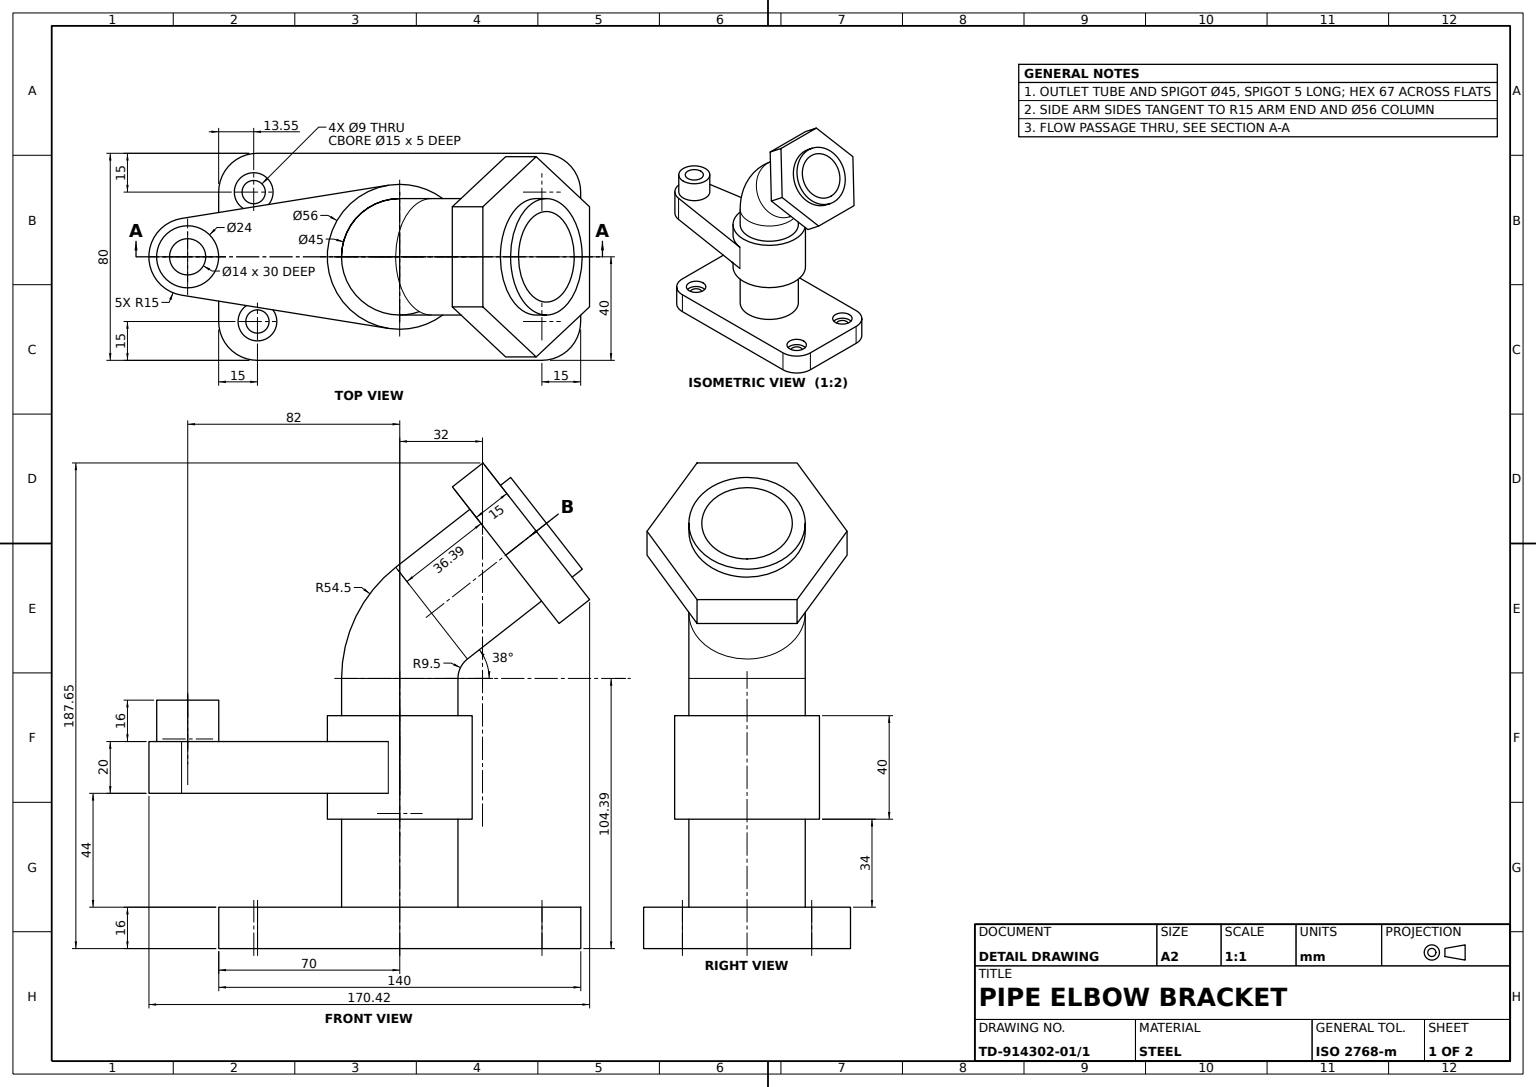
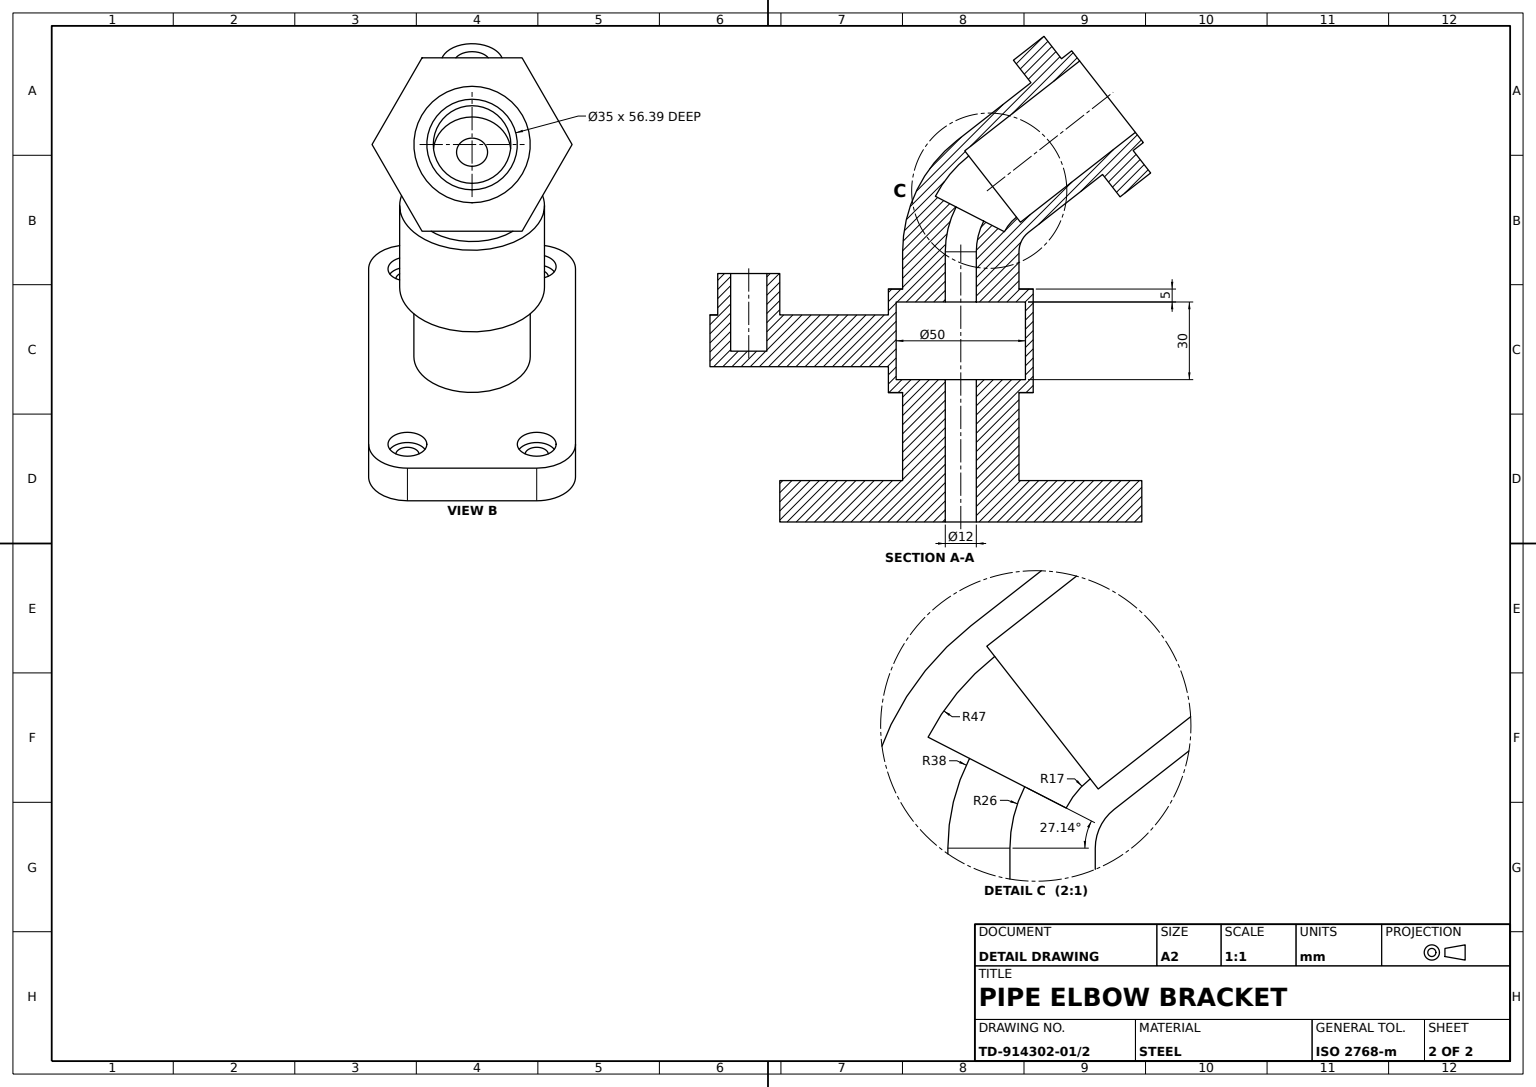
solid
v1 (-55,11,17.5)
v2 (-55,16,17.5)
e1 v1 v2 LINE
v3 (-55,16,32.5)
e2 v2 v3 CIRCLE(AX(P(-55,16,25),D(0,1,0),D(0,0,1)),7.5)
v4 (-55,11,32.5)
e3 v4 v3 LINE
e4 v1 v4 CIRCLE(AX(P(-55,11,25),D(0,1,0),D(0,0,1)),7.5)
face CYL(AX(P(-55,16,25),D(0,1,0),D(0,0,1)),7.5) rev [e1 e2 -e3 -e4]
v5 (61.601219,125.616036,19.341234)
v6 (73.42138,134.850959,19.341234)
e5 v5 v6 LINE
v7 (61.601219,125.616036,-19.341234)
e6 v5 v7 LINE
v8 (73.42138,134.850959,-19.341234)
e7 v7 v8 LINE
e8 v6 v8 LINE
face PLANE(AX(P(61.601219,125.616036,19.341234),D(0.615661475,-0.788010754,0),D(0.788010754,0.615661475,0))) [-e5 e6 e7 -e8]
v9 (-82,80,-12)
v10 (-82,80,12)
e9 v9 v10 CIRCLE(AX(P(-82,80,0),D(0,1,0),D(0,0,1)),12)
v11 (-82,96,12)
e10 v11 v10 LINE
v12 (-82,96,-12)
e11 v12 v11 CIRCLE(AX(P(-82,96,0),D(0,1,0),D(0,0,1)),12)
e12 v12 v9 LINE
face CYL(AX(P(-82,96,0),D(0,-1,0),D(0,0,-1)),12) [e9 -e10 -e11 e12]
v13 (55,11,17.5)
v14 (55,16,17.5)
e13 v13 v14 LINE
v15 (55,11,32.5)
e14 v15 v13 CIRCLE(AX(P(55,11,25),D(0,1,0),D(0,0,1)),7.5)
v16 (55,16,32.5)
e15 v15 v16 LINE
e16 v16 v14 CIRCLE(AX(P(55,16,25),D(0,1,0),D(0,0,1)),7.5)
face CYL(AX(P(55,16,25),D(0,1,0),D(0,0,1)),7.5) rev [-e13 -e14 e15 e16]
v17 (0,90,22.5)
v18 (0,90,-22.5)
e17 v17 v18 CIRCLE(AX(P(0,90,0),D(0,-1,0),D(0,0,1)),22.5)
v19 (0,104.392557,22.5)
e18 v17 v19 LINE
v20 (-22.5,104.392557,0)
e19 v19 v20 CIRCLE(AX(P(0,104.392557,0),D(0,-1,0),D(1,0,0)),22.5)
v21 (0,104.392557,-22.5)
e20 v20 v21 CIRCLE(AX(P(0,104.392557,0),D(0,-1,0),D(1,0,0)),22.5)
e21 v18 v21 LINE
face CYL(AX(P(0,0,0),D(0,1,0),D(0,0,1)),22.5) [-e17 e18 e19 e20 -e21]
v22 (0,0,6)
v23 (0,0,-6)
e22 v22 v23 CIRCLE(AX(P(0,0,0),D(0,-1,0),D(0,0,-1)),6)
v24 (0,55,-6)
e23 v23 v24 LINE
v25 (0,55,6)
e24 v24 v25 CIRCLE(AX(P(0,55,0),D(0,1,0),D(0,0,1)),6)
e25 v22 v25 LINE
face CYL(AX(P(0,-1.043926,0),D(0,1,0),D(0,0,1)),6) rev [e22 e23 e24 -e25]
v26 (27.124176,169.744639,0)
v27 (54.828942,134.284155,0)
e26 v26 v27 CIRCLE(AX(P(40.976559,152.014397,0),D(0.788010754,0.615661475,0),D(-0.615661475,0.788010754,0)),22.5)
e27 v27 v26 CIRCLE(AX(P(40.976559,152.014397,0),D(0.788010754,0.615661475,0),D(-0.615661475,0.788010754,0)),22.5)
v28 (20.3519,178.412757,19.341234)
v29 (40.976559,152.014397,38.682468)
e28 v28 v29 LINE
v30 (20.3519,178.412757,-19.341234)
e29 v30 v28 LINE
v31 (40.976559,152.014397,-38.682468)
e30 v31 v30 LINE
e31 v7 v31 LINE
e32 v29 v5 LINE
face PLANE(AX(P(99.194303,77.499083,0),D(0.788010754,0.615661475,0),D(-0.615661475,0.788010754,0))) rev [e26 e27] [-e28 -e29 -e30 -e31 -e6 -e32]
v32 (70,16,25)
v33 (70,16,-25)
e33 v32 v33 LINE
v34 (70,0,25)
e34 v32 v34 LINE
v35 (70,0,-25)
e35 v34 v35 LINE
e36 v35 v33 LINE
face PLANE(AX(P(70,16,40),D(-1,0,0),D(0,0,1))) rev [-e33 e34 e35 e36]
v36 (-56.445631,0,-29.5)
v37 (-56.445631,11,-29.5)
e37 v36 v37 LINE
v38 (-56.445631,0,-20.5)
e38 v36 v38 CIRCLE(AX(P(-56.445631,0,-25),D(0,-1,0),D(0,0,-1)),4.5)
v39 (-56.445631,11,-20.5)
e39 v38 v39 LINE
e40 v39 v37 CIRCLE(AX(P(-56.445631,11,-25),D(0,1,0),D(0,0,1)),4.5)
face CYL(AX(P(-56.445631,16,-25),D(0,1,0),D(0,0,1)),4.5) rev [-e37 e38 e39 e40]
v40 (52.79672,161.249319,38.682468)
e41 v40 v6 LINE
e42 v29 v40 LINE
face PLANE(AX(P(40.976559,152.014397,38.682468),D(0.307830738,-0.394005377,0.866025404),D(0,-0.91022489,-0.414114296))) [e5 -e41 -e42 e32]
v41 (55,11,29.5)
v42 (55,11,20.5)
e43 v41 v42 CIRCLE(AX(P(55,11,25),D(0,1,0),D(0,0,1)),4.5)
e44 v42 v41 CIRCLE(AX(P(55,11,25),D(0,1,0),D(0,0,1)),4.5)
e45 v13 v15 CIRCLE(AX(P(55,11,25),D(0,1,0),D(0,0,1)),7.5)
face PLANE(AX(P(59.5,11,25),D(0,-1,0),D(0,0,-1))) rev [-e43 -e44] [e45 e14]
v43 (-84.378049,60,14.810297)
v44 (-4.439024,60,27.645887)
e46 v43 v44 LINE
v45 (-84.378049,60,-14.810297)
e47 v45 v43 CIRCLE(AX(P(-82,60,0),D(0,1,0),D(0,0,1)),15)
v46 (-4.439024,60,-27.645887)
e48 v46 v45 LINE
e49 v44 v46 CIRCLE(AX(P(0,60,0),D(0,-1,0),D(0,0,1)),28)
face PLANE(AX(P(-82,60,0),D(0,1,0),D(0,0,1))) rev [-e46 -e47 -e48 -e49]
v47 (55,11,-17.5)
v48 (55,16,-17.5)
e50 v47 v48 LINE
v49 (55,16,-32.5)
e51 v48 v49 CIRCLE(AX(P(55,16,-25),D(0,1,0),D(0,0,1)),7.5)
v50 (55,11,-32.5)
e52 v50 v49 LINE
e53 v47 v50 CIRCLE(AX(P(55,11,-25),D(0,1,0),D(0,0,1)),7.5)
face CYL(AX(P(55,16,-25),D(0,1,0),D(0,0,1)),7.5) rev [e50 e51 -e52 -e53]
v51 (55,16,40)
e54 v51 v32 CIRCLE(AX(P(55,16,25),D(0,1,0),D(0,0,-1)),15)
v52 (55,0,40)
e55 v52 v51 LINE
e56 v34 v52 CIRCLE(AX(P(55,0,25),D(0,-1,0),D(0,0,-1)),15)
face CYL(AX(P(55,16,25),D(0,-1,0),D(0,0,-1)),15) [-e54 -e55 -e56 -e34]
v53 (0,55,-25)
v54 (0,55,25)
e57 v53 v54 CIRCLE(AX(P(0,55,0),D(0,-1,0),D(0,0,-1)),25)
e58 v54 v53 CIRCLE(AX(P(0,55,0),D(0,-1,0),D(0,0,-1)),25)
e59 v25 v24 CIRCLE(AX(P(0,55,0),D(0,1,0),D(0,0,1)),6)
face PLANE(AX(P(-25,55,0),D(0,1,0),D(0,0,1))) [-e57 -e58] [-e24 -e59]
e60 v10 v9 CIRCLE(AX(P(-82,80,0),D(0,1,0),D(0,0,1)),12)
e61 v11 v12 CIRCLE(AX(P(-82,96,0),D(0,1,0),D(0,0,1)),12)
face CYL(AX(P(-82,96,0),D(0,-1,0),D(0,0,-1)),12) [e10 e60 -e12 -e61]
v55 (-4.439024,80,27.645887)
v56 (-4.439024,80,-27.645887)
e62 v55 v56 CIRCLE(AX(P(0,80,0),D(0,-1,0),D(0,0,1)),28)
e63 v55 v44 LINE
e64 v56 v46 LINE
v57 (0,90,28)
v58 (0,50,28)
e65 v57 v58 LINE
v59 (0,90,-28)
e66 v59 v57 CIRCLE(AX(P(0,90,0),D(0,1,0),D(0,0,1)),28)
v60 (0,50,-28)
e67 v59 v60 LINE
e68 v60 v58 CIRCLE(AX(P(0,50,0),D(0,1,0),D(0,0,1)),28)
face CYL(AX(P(0,90,0),D(0,-1,0),D(0,0,-1)),28) [-e62 e63 e49 -e64] [-e65 -e66 e67 e68]
v61 (-84.378049,80,-14.810297)
e69 v56 v61 LINE
e70 v61 v45 LINE
face PLANE(AX(P(-84.378049,80,-14.810297),D(0.158536585,0,0.987353104),D(0.987353104,0,-0.158536585))) rev [-e69 e64 e48 -e70]
v62 (0,85,25)
v63 (0,85,-25)
e71 v62 v63 CIRCLE(AX(P(0,85,0),D(0,-1,0),D(0,0,-1)),25)
e72 v62 v54 LINE
e73 v63 v53 LINE
face CYL(AX(P(0,55,0),D(0,-1,0),D(0,0,-1)),25) rev [-e71 e72 e58 -e73]
e74 v57 v59 CIRCLE(AX(P(0,90,0),D(0,1,0),D(0,0,1)),28)
e75 v58 v60 CIRCLE(AX(P(0,50,0),D(0,1,0),D(0,0,1)),28)
face CYL(AX(P(0,90,0),D(0,-1,0),D(0,0,-1)),28) [-e74 e65 e75 -e67]
v64 (32.172061,187.647679,-19.341234)
e76 v30 v64 LINE
v65 (32.172061,187.647679,19.341234)
e77 v28 v65 LINE
e78 v64 v65 LINE
face PLANE(AX(P(20.3519,178.412757,-19.341234),D(-0.615661475,0.788010754,0),D(-0.788010754,-0.615661475,0))) [-e76 e29 e77 -e78]
v66 (-55,16,40)
v67 (-55,0,40)
e79 v66 v67 LINE
e80 v67 v52 LINE
e81 v66 v51 LINE
face PLANE(AX(P(-70,16,40),D(0,0,-1),D(-1,0,0))) rev [e79 e80 e55 -e81]
e82 v38 v36 CIRCLE(AX(P(-56.445631,0,-25),D(0,-1,0),D(0,0,-1)),4.5)
v68 (-55,0,20.5)
v69 (-55,0,29.5)
e83 v68 v69 CIRCLE(AX(P(-55,0,25),D(0,-1,0),D(0,0,-1)),4.5)
e84 v69 v68 CIRCLE(AX(P(-55,0,25),D(0,-1,0),D(0,0,-1)),4.5)
v70 (55,0,-29.5)
v71 (55,0,-20.5)
e85 v70 v71 CIRCLE(AX(P(55,0,-25),D(0,-1,0),D(0,0,-1)),4.5)
e86 v71 v70 CIRCLE(AX(P(55,0,-25),D(0,-1,0),D(0,0,-1)),4.5)
v72 (55,0,-40)
v73 (-55,0,-40)
e87 v72 v73 LINE
e88 v72 v35 CIRCLE(AX(P(55,0,-25),D(0,-1,0),D(0,0,-1)),15)
v74 (-70,0,25)
e89 v67 v74 CIRCLE(AX(P(-55,0,25),D(0,-1,0),D(0,0,-1)),15)
v75 (-70,0,-25)
e90 v75 v74 LINE
e91 v75 v73 CIRCLE(AX(P(-55,0,-25),D(0,-1,0),D(0,0,-1)),15)
v76 (55,0,29.5)
v77 (55,0,20.5)
e92 v76 v77 CIRCLE(AX(P(55,0,25),D(0,-1,0),D(0,0,-1)),4.5)
e93 v77 v76 CIRCLE(AX(P(55,0,25),D(0,-1,0),D(0,0,-1)),4.5)
e94 v23 v22 CIRCLE(AX(P(0,0,0),D(0,-1,0),D(0,0,-1)),6)
face PLANE(AX(P(0,0,0),D(0,-1,0),D(0,0,-1))) [-e38 -e82] [-e83 -e84] [-e85 -e86] [-e87 e88 -e35 e56 -e80 e89 -e90 e91] [-e92 -e93] [-e22 -e94]
v78 (52.79672,161.249319,-38.682468)
e95 v31 v78 LINE
e96 v8 v78 LINE
face PLANE(AX(P(61.601219,125.616036,-19.341234),D(0.307830738,-0.394005377,-0.866025404),D(0,0.91022489,-0.414114296))) [e95 -e96 -e7 e31]
v79 (-55,16,-40)
e97 v73 v79 LINE
v80 (-70,16,-25)
e98 v80 v75 LINE
e99 v79 v80 CIRCLE(AX(P(-55,16,-25),D(0,1,0),D(0,0,-1)),15)
face CYL(AX(P(-55,16,-25),D(0,-1,0),D(0,0,-1)),15) [-e97 -e91 -e98 -e99]
v81 (-84.378049,80,14.810297)
e100 v81 v43 LINE
e101 v81 v55 LINE
face PLANE(AX(P(-84.378049,80,14.810297),D(0.158536585,0,-0.987353104),D(-0.987353104,0,-0.158536585))) rev [e100 e46 -e63 -e101]
v82 (16.871748,112.147296,0)
v83 (-9.825169,125.83213,0)
e102 v82 v83 CIRCLE(AX(P(3.523289,118.989713,0),D(0.45616112,0.889897204,0),D(-0.889897204,0.45616112,0)),15)
e103 v83 v82 CIRCLE(AX(P(3.523289,118.989713,0),D(0.45616112,0.889897204,0),D(-0.889897204,0.45616112,0)),15)
v84 (8.862673,116.252746,0)
v85 (-1.816094,121.72668,0)
e104 v84 v85 CIRCLE(AX(P(3.523289,118.989713,0),D(-0.45616112,-0.889897204,0),D(-0.889897204,0.45616112,0)),6)
e105 v85 v84 CIRCLE(AX(P(3.523289,118.989713,0),D(-0.45616112,-0.889897204,0),D(-0.889897204,0.45616112,0)),6)
face PLANE(AX(P(3.523289,118.989713,0),D(0.45616112,0.889897204,0),D(-0.889897204,0.45616112,0))) [e102 e103] [e104 e105]
e106 v4 v1 CIRCLE(AX(P(-55,11,25),D(0,1,0),D(0,0,1)),7.5)
v86 (-55,11,29.5)
v87 (-55,11,20.5)
e107 v86 v87 CIRCLE(AX(P(-55,11,25),D(0,1,0),D(0,0,1)),4.5)
e108 v87 v86 CIRCLE(AX(P(-55,11,25),D(0,1,0),D(0,0,1)),4.5)
face PLANE(AX(P(-50.5,11,25),D(0,-1,0),D(0,0,-1))) rev [e106 e4] [-e107 -e108]
e109 v68 v87 LINE
e110 v69 v86 LINE
face CYL(AX(P(-55,16,25),D(0,1,0),D(0,0,1)),4.5) rev [e84 e109 e108 -e110]
v88 (-1.55355,147.339143,0)
v89 (26.151216,111.878659,0)
e111 v88 v89 CIRCLE(AX(P(12.298833,129.608901,0),D(-0.788010754,-0.615661475,0),D(0.615661475,-0.788010754,0)),22.5)
v90 (22.5,104.392557,0)
e112 v90 v89 CIRCLE(AX(P(32,104.392557,0),D(0,0,-1),D(-1,0,0)),9.5)
e113 v21 v90 CIRCLE(AX(P(0,104.392557,0),D(0,-1,0),D(1,0,0)),22.5)
e114 v20 v88 CIRCLE(AX(P(32,104.392557,0),D(0,0,-1),D(-1,0,0)),54.5)
face TORUS(AX(P(32,104.392557,0),D(0,0,-1),D(-1,0,0)),32,22.5) [e111 -e112 -e113 -e20 e114]
v91 (21.533755,117.78874,0)
e115 v91 v82 CIRCLE(AX(P(32,104.392557,0),D(0,0,1),D(1,0,0)),17)
v92 (3.063911,141.429063,0)
e116 v92 v83 CIRCLE(AX(P(32,104.392557,0),D(0,0,1),D(1,0,0)),47)
e117 v92 v91 CIRCLE(AX(P(12.298833,129.608901,0),D(0.788010754,0.615661475,0),D(-0.615661475,0.788010754,0)),15)
face TORUS(AX(P(32,104.392557,0),D(0,0,1),D(1,0,0)),32,15) rev [e115 -e103 -e116 e117]
e118 v61 v81 CIRCLE(AX(P(-82,80,0),D(0,1,0),D(0,0,1)),15)
face CYL(AX(P(-82,80,0),D(0,-1,0),D(0,0,-1)),15) [-e100 -e118 e70 e47]
e119 v77 v42 LINE
e120 v76 v41 LINE
face CYL(AX(P(55,16,25),D(0,1,0),D(0,0,1)),4.5) rev [e119 e44 -e120 e92]
e121 v63 v62 CIRCLE(AX(P(0,85,0),D(0,-1,0),D(0,0,-1)),25)
face CYL(AX(P(0,55,0),D(0,-1,0),D(0,0,-1)),25) rev [e73 e57 -e72 -e121]
v93 (55,16,-40)
e122 v93 v72 LINE
e123 v33 v93 CIRCLE(AX(P(55,16,-25),D(0,1,0),D(0,0,-1)),15)
face CYL(AX(P(55,16,-25),D(0,-1,0),D(0,0,-1)),15) [-e122 -e123 -e36 -e88]
v94 (55,11,-20.5)
v95 (55,11,-29.5)
e124 v94 v95 CIRCLE(AX(P(55,11,-25),D(0,1,0),D(0,0,1)),4.5)
e125 v95 v94 CIRCLE(AX(P(55,11,-25),D(0,1,0),D(0,0,1)),4.5)
e126 v50 v47 CIRCLE(AX(P(55,11,-25),D(0,1,0),D(0,0,1)),7.5)
face PLANE(AX(P(59.5,11,-25),D(0,-1,0),D(0,0,-1))) rev [-e124 -e125] [e53 e126]
v96 (-82,66,-7)
v97 (-82,66,7)
e127 v96 v97 CIRCLE(AX(P(-82,66,0),D(0,1,0),D(0,0,1)),7)
e128 v97 v96 CIRCLE(AX(P(-82,66,0),D(0,1,0),D(0,0,1)),7)
face PLANE(AX(P(-82,66,0),D(0,1,0),D(0,0,1))) [e127 e128]
v98 (-82,96,-7)
e129 v96 v98 LINE
v99 (-82,96,7)
e130 v97 v99 LINE
e131 v99 v98 CIRCLE(AX(P(-82,96,0),D(0,1,0),D(0,0,1)),7)
face CYL(AX(P(-82,66,0),D(0,1,0),D(0,0,1)),7) rev [-e129 -e128 e130 e131]
e132 v98 v99 CIRCLE(AX(P(-82,96,0),D(0,1,0),D(0,0,1)),7)
face PLANE(AX(P(-82,96,0),D(0,1,0),D(0,0,1))) [e11 e61] [-e131 -e132]
face CYL(AX(P(0,-1.043926,0),D(0,1,0),D(0,0,1)),6) rev [e25 e59 -e23 e94]
face CYL(AX(P(-82,66,0),D(0,1,0),D(0,0,1)),7) rev [-e127 e129 e132 -e130]
v100 (23.072909,115.818713,0)
v101 (1.524757,143.399089,0)
e133 v100 v101 CIRCLE(AX(P(12.298833,129.608901,0),D(0.788010754,0.615661475,0),D(-0.615661475,0.788010754,0)),17.5)
v102 (67.51085,150.537438,0)
e134 v100 v102 LINE
v103 (45.962698,178.117814,0)
e135 v102 v103 CIRCLE(AX(P(56.736774,164.327626,0),D(0.788010754,0.615661475,0),D(-0.615661475,0.788010754,0)),17.5)
e136 v101 v103 LINE
face CYL(AX(P(12.298833,129.608901,0),D(0.788010754,0.615661475,0),D(-0.615661475,0.788010754,0)),17.5) rev [-e133 e134 e135 -e136]
e137 v88 v26 LINE
e138 v89 v27 LINE
face CYL(AX(P(12.298833,129.608901,0),D(0.788010754,0.615661475,0),D(-0.615661475,0.788010754,0)),22.5) [-e111 e137 -e27 -e138]
v104 (0,104.392557,-6)
v105 (6,104.392557,0)
e139 v104 v105 CIRCLE(AX(P(0,104.392557,0),D(0,-1,0),D(1,0,0)),6)
e140 v105 v84 CIRCLE(AX(P(32,104.392557,0),D(0,0,-1),D(-1,0,0)),26)
v106 (-6,104.392557,0)
e141 v106 v85 CIRCLE(AX(P(32,104.392557,0),D(0,0,-1),D(-1,0,0)),38)
e142 v106 v104 CIRCLE(AX(P(0,104.392557,0),D(0,-1,0),D(1,0,0)),6)
face TORUS(AX(P(32,104.392557,0),D(0,0,-1),D(-1,0,0)),32,6) rev [e139 e140 -e105 -e141 e142]
e143 v49 v48 CIRCLE(AX(P(55,16,-25),D(0,1,0),D(0,0,1)),7.5)
e144 v3 v2 CIRCLE(AX(P(-55,16,25),D(0,1,0),D(0,0,1)),7.5)
e145 v14 v16 CIRCLE(AX(P(55,16,25),D(0,1,0),D(0,0,1)),7.5)
v107 (-70,16,25)
e146 v107 v66 CIRCLE(AX(P(-55,16,25),D(0,1,0),D(0,0,-1)),15)
e147 v93 v79 LINE
e148 v80 v107 LINE
v108 (-56.445631,16,-17.5)
v109 (-56.445631,16,-32.5)
e149 v108 v109 CIRCLE(AX(P(-56.445631,16,-25),D(0,1,0),D(0,0,1)),7.5)
e150 v109 v108 CIRCLE(AX(P(-56.445631,16,-25),D(0,1,0),D(0,0,1)),7.5)
v110 (0,16,-22.5)
v111 (0,16,22.5)
e151 v110 v111 CIRCLE(AX(P(0,16,0),D(0,1,0),D(0,0,1)),22.5)
e152 v111 v110 CIRCLE(AX(P(0,16,0),D(0,1,0),D(0,0,1)),22.5)
face PLANE(AX(P(0,16,0),D(0,-1,0),D(0,0,-1))) rev [-e143 -e51] [-e2 -e144] [-e145 -e16] [e146 e81 e54 e33 e123 e147 e99 e148] [-e149 -e150] [-e151 -e152]
e153 v91 v92 CIRCLE(AX(P(12.298833,129.608901,0),D(0.788010754,0.615661475,0),D(-0.615661475,0.788010754,0)),15)
face TORUS(AX(P(32,104.392557,0),D(0,0,1),D(1,0,0)),32,15) rev [-e115 e153 e116 -e102]
e154 v37 v39 CIRCLE(AX(P(-56.445631,11,-25),D(0,1,0),D(0,0,1)),4.5)
face CYL(AX(P(-56.445631,16,-25),D(0,1,0),D(0,0,1)),4.5) rev [e154 -e39 e82 e37]
e155 v71 v94 LINE
e156 v70 v95 LINE
face CYL(AX(P(55,16,-25),D(0,1,0),D(0,0,1)),4.5) rev [-e155 e86 e156 e125]
face CYL(AX(P(55,16,-25),D(0,1,0),D(0,0,1)),4.5) rev [-e156 e85 e155 e124]
e157 v103 v102 CIRCLE(AX(P(56.736774,164.327626,0),D(0.788010754,0.615661475,0),D(-0.615661475,0.788010754,0)),17.5)
v112 (70.589157,146.597384,0)
v113 (42.884391,182.057868,0)
e158 v112 v113 CIRCLE(AX(P(56.736774,164.327626,0),D(-0.788010754,-0.615661475,0),D(0.615661475,-0.788010754,0)),22.5)
e159 v113 v112 CIRCLE(AX(P(56.736774,164.327626,0),D(-0.788010754,-0.615661475,0),D(0.615661475,-0.788010754,0)),22.5)
face PLANE(AX(P(56.736774,164.327626,0),D(-0.788010754,-0.615661475,0),D(0.615661475,-0.788010754,0))) rev [-e157 -e135] [-e158 -e159]
e160 v90 v19 CIRCLE(AX(P(0,104.392557,0),D(0,-1,0),D(1,0,0)),22.5)
e161 v18 v17 CIRCLE(AX(P(0,90,0),D(0,-1,0),D(0,0,1)),22.5)
face CYL(AX(P(0,0,0),D(0,1,0),D(0,0,1)),22.5) [e21 e113 e160 -e18 -e161]
v114 (0,85,-6)
e162 v114 v104 LINE
v115 (0,85,6)
e163 v114 v115 CIRCLE(AX(P(0,85,0),D(0,-1,0),D(0,0,-1)),6)
v116 (0,104.392557,6)
e164 v115 v116 LINE
e165 v105 v116 CIRCLE(AX(P(0,104.392557,0),D(0,-1,0),D(1,0,0)),6)
face CYL(AX(P(0,-1.043926,0),D(0,1,0),D(0,0,1)),6) rev [-e139 -e162 e163 e164 -e165]
v117 (-56.445631,11,-17.5)
v118 (-56.445631,11,-32.5)
e166 v117 v118 CIRCLE(AX(P(-56.445631,11,-25),D(0,1,0),D(0,0,1)),7.5)
e167 v117 v108 LINE
e168 v118 v109 LINE
face CYL(AX(P(-56.445631,16,-25),D(0,1,0),D(0,0,1)),7.5) rev [-e166 e167 e149 -e168]
e169 v101 v100 CIRCLE(AX(P(12.298833,129.608901,0),D(0.788010754,0.615661475,0),D(-0.615661475,0.788010754,0)),17.5)
face PLANE(AX(P(12.298833,129.608901,0),D(0.788010754,0.615661475,0),D(-0.615661475,0.788010754,0))) [-e153 -e117] [e133 e169]
face CYL(AX(P(55,16,25),D(0,1,0),D(0,0,1)),4.5) rev [e43 -e119 e93 e120]
e170 v74 v107 LINE
face CYL(AX(P(-55,16,25),D(0,-1,0),D(0,0,-1)),15) [-e170 -e89 -e79 -e146]
face PLANE(AX(P(-82,80,0),D(0,1,0),D(0,0,1))) [e69 e118 e101 e62] [-e60 -e9]
e171 v115 v114 CIRCLE(AX(P(0,85,0),D(0,-1,0),D(0,0,-1)),6)
e172 v116 v106 CIRCLE(AX(P(0,104.392557,0),D(0,-1,0),D(1,0,0)),6)
face CYL(AX(P(0,-1.043926,0),D(0,1,0),D(0,0,1)),6) rev [-e164 e171 e162 -e142 -e172]
face CYL(AX(P(55,16,-25),D(0,1,0),D(0,0,1)),7.5) rev [e52 e143 -e50 -e126]
v119 (66.649104,143.519077,0)
e173 v119 v112 LINE
v120 (38.944337,178.979561,0)
e174 v119 v120 CIRCLE(AX(P(52.79672,161.249319,0),D(0.788010754,0.615661475,0),D(-0.615661475,0.788010754,0)),22.5)
e175 v120 v113 LINE
face CYL(AX(P(12.298833,129.608901,0),D(0.788010754,0.615661475,0),D(-0.615661475,0.788010754,0)),22.5) [-e173 e174 e175 e159]
e176 v89 v88 CIRCLE(AX(P(12.298833,129.608901,0),D(-0.788010754,-0.615661475,0),D(0.615661475,-0.788010754,0)),22.5)
face CYL(AX(P(12.298833,129.608901,0),D(0.788010754,0.615661475,0),D(-0.615661475,0.788010754,0)),22.5) [e138 -e26 -e137 -e176]
e177 v120 v119 CIRCLE(AX(P(52.79672,161.249319,0),D(0.788010754,0.615661475,0),D(-0.615661475,0.788010754,0)),22.5)
e178 v78 v64 LINE
e179 v65 v40 LINE
face PLANE(AX(P(111.014464,86.734005,0),D(0.788010754,0.615661475,0),D(-0.615661475,0.788010754,0))) [-e177 -e174] [e8 e96 e178 e78 e179 e41]
face CYL(AX(P(-55,16,25),D(0,1,0),D(0,0,1)),4.5) rev [-e109 e83 e110 e107]
face PLANE(AX(P(-70,16,-40),D(0,0,1),D(1,0,0))) rev [e97 -e147 e122 e87]
face CYL(AX(P(12.298833,129.608901,0),D(0.788010754,0.615661475,0),D(-0.615661475,0.788010754,0)),22.5) [e177 e173 e158 -e175]
v121 (0,50,-22.5)
e180 v121 v110 LINE
v122 (0,50,22.5)
e181 v122 v111 LINE
e182 v121 v122 CIRCLE(AX(P(0,50,0),D(0,1,0),D(0,0,1)),22.5)
face CYL(AX(P(0,50,0),D(0,-1,0),D(0,0,-1)),22.5) [e180 e151 -e181 -e182]
face CYL(AX(P(55,16,25),D(0,1,0),D(0,0,1)),7.5) rev [-e15 -e45 e13 e145]
e183 v122 v121 CIRCLE(AX(P(0,50,0),D(0,1,0),D(0,0,1)),22.5)
face CYL(AX(P(0,50,0),D(0,-1,0),D(0,0,-1)),22.5) [e152 -e180 -e183 e181]
e184 v118 v117 CIRCLE(AX(P(-56.445631,11,-25),D(0,1,0),D(0,0,1)),7.5)
face PLANE(AX(P(-51.945631,11,-25),D(0,-1,0),D(0,0,-1))) rev [-e154 -e40] [e184 e166]
face TORUS(AX(P(32,104.392557,0),D(0,0,-1),D(-1,0,0)),32,22.5) [-e160 e112 e176 -e114 -e19]
face CYL(AX(P(-55,16,25),D(0,1,0),D(0,0,1)),7.5) rev [-e106 e3 e144 -e1]
face PLANE(AX(P(40.976559,152.014397,-38.682468),D(-0.307830738,0.394005377,-0.866025404),D(0,0.91022489,0.414114296))) [-e95 e30 e76 -e178]
face PLANE(AX(P(20.3519,178.412757,19.341234),D(-0.307830738,0.394005377,0.866025404),D(0,-0.91022489,0.414114296))) [-e77 e28 e42 -e179]
face TORUS(AX(P(32,104.392557,0),D(0,0,-1),D(-1,0,0)),32,6) rev [e165 e172 e141 -e104 -e140]
face PLANE(AX(P(0,50,0),D(0,1,0),D(0,0,1))) rev [e183 e182] [-e68 -e75]
face PLANE(AX(P(0,90,0),D(0,1,0),D(0,0,1))) [e161 e17] [e66 e74]
face PLANE(AX(P(0,85,0),D(0,-1,0),D(0,0,-1))) [e121 e71] [-e163 -e171]
face PLANE(AX(P(-70,16,40),D(1,0,0),D(0,0,-1))) rev [e170 -e148 e98 e90]
face CYL(AX(P(12.298833,129.608901,0),D(0.788010754,0.615661475,0),D(-0.615661475,0.788010754,0)),17.5) rev [-e169 e136 e157 -e134]
face CYL(AX(P(-56.445631,16,-25),D(0,1,0),D(0,0,1)),7.5) rev [-e184 e168 e150 -e167]
